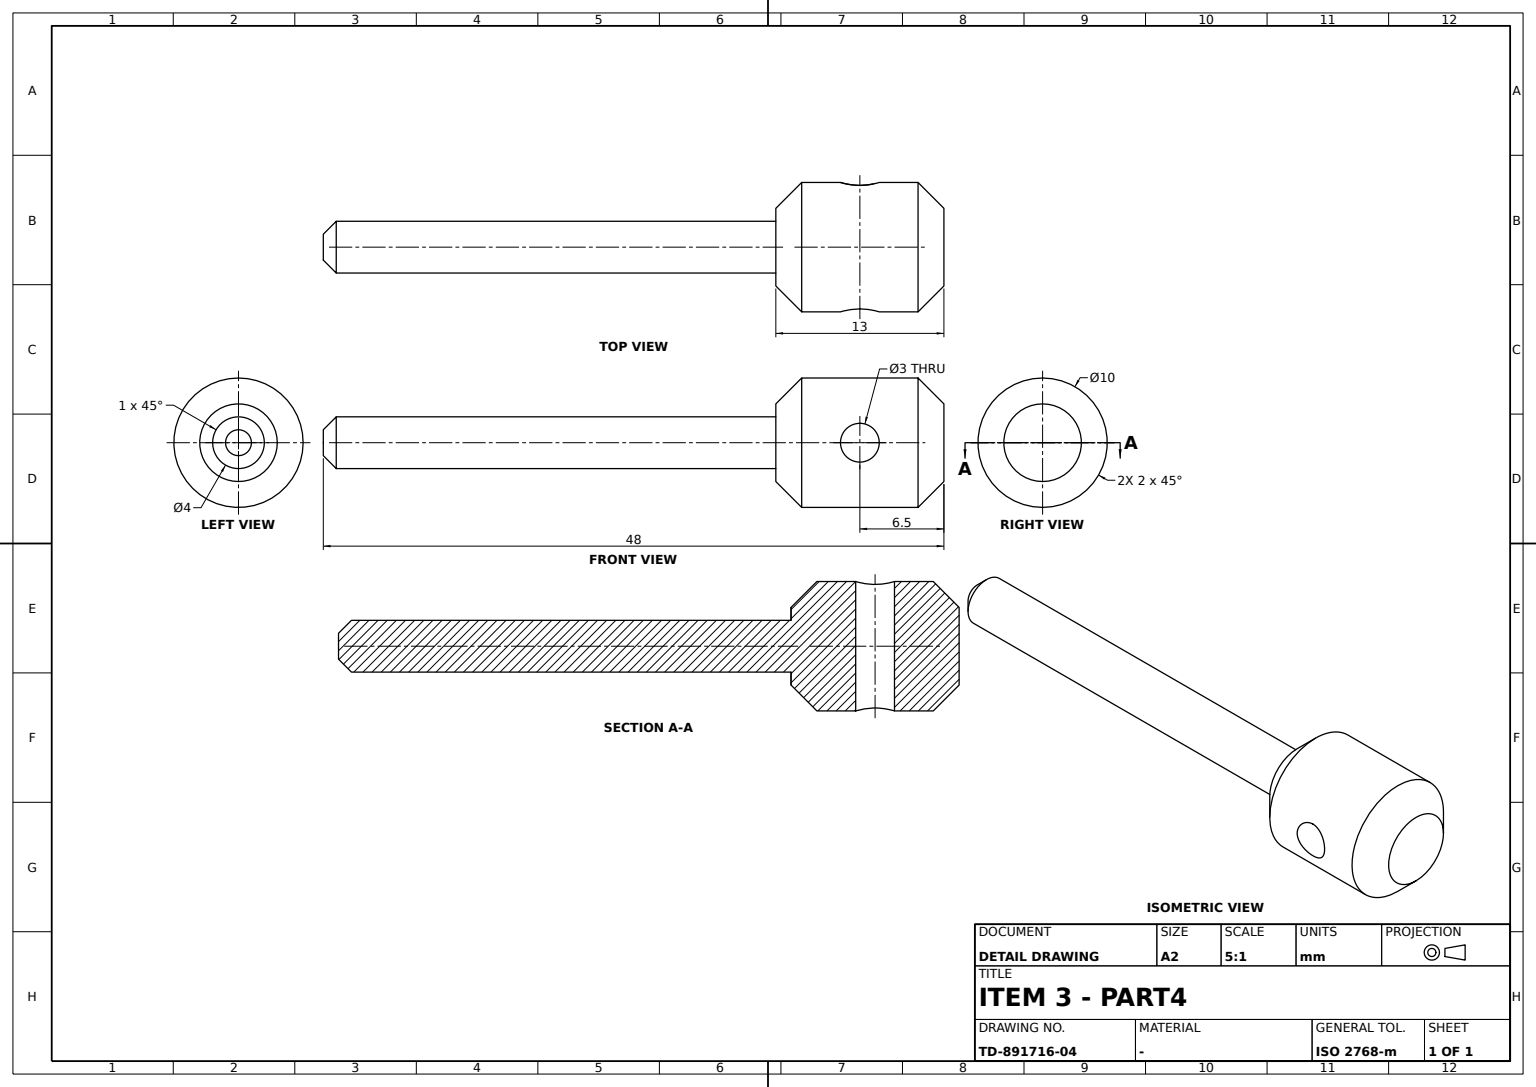
ISO-10303-21;
HEADER;
FILE_DESCRIPTION((''),'2;1');
FILE_NAME('','',(''),(''),'','','');
FILE_SCHEMA(('AUTOMOTIVE_DESIGN'));
ENDSEC;
DATA;
#1=APPLICATION_CONTEXT('');
#2=PRODUCT_CONTEXT('',#1,'mechanical');
#3=PRODUCT('','','',(#2));
#4=PRODUCT_DEFINITION_FORMATION('','',#3);
#5=PRODUCT_DEFINITION_CONTEXT('',#1,'design');
#6=PRODUCT_DEFINITION('','',#4,#5);
#7=PRODUCT_DEFINITION_SHAPE('','',#6);
#8=(LENGTH_UNIT()NAMED_UNIT(*)SI_UNIT(.MILLI.,.METRE.));
#9=(NAMED_UNIT(*)PLANE_ANGLE_UNIT()SI_UNIT($,.RADIAN.));
#10=(NAMED_UNIT(*)SI_UNIT($,.STERADIAN.)SOLID_ANGLE_UNIT());
#11=UNCERTAINTY_MEASURE_WITH_UNIT(LENGTH_MEASURE(0.005),#8,'distance_accuracy_value','');
#12=(GEOMETRIC_REPRESENTATION_CONTEXT(3)GLOBAL_UNCERTAINTY_ASSIGNED_CONTEXT((#11))GLOBAL_UNIT_ASSIGNED_CONTEXT((#8,#9,#10))REPRESENTATION_CONTEXT('',''));
#13=CARTESIAN_POINT('',(0.,-5.,2.));
#14=VERTEX_POINT('',#13);
#15=CARTESIAN_POINT('',(0.,0.,2.));
#16=DIRECTION('',(0.,0.,1.));
#17=DIRECTION('',(0.,-1.,0.));
#18=AXIS2_PLACEMENT_3D('',#15,#16,#17);
#19=CIRCLE('',#18,5.);
#20=EDGE_CURVE('',#14,#14,#19,.T.);
#21=ORIENTED_EDGE('',*,*,#20,.T.);
#22=EDGE_LOOP('',(#21));
#23=FACE_BOUND('',#22,.T.);
#24=CARTESIAN_POINT('',(-5.,0.,11.));
#25=VERTEX_POINT('',#24);
#26=CARTESIAN_POINT('',(0.,0.,11.));
#27=DIRECTION('',(0.,0.,-1.));
#28=DIRECTION('',(-1.,0.,0.));
#29=AXIS2_PLACEMENT_3D('',#26,#27,#28);
#30=CIRCLE('',#29,5.);
#31=EDGE_CURVE('',#25,#25,#30,.F.);
#32=ORIENTED_EDGE('',*,*,#31,.F.);
#33=EDGE_LOOP('',(#32));
#34=FACE_BOUND('',#33,.T.);
#35=CARTESIAN_POINT('',(-1.5,-4.769696,6.5));
#36=VERTEX_POINT('',#35);
#37=CARTESIAN_POINT('',(-1.175074,-4.887685,7.676025));
#38=CARTESIAN_POINT('',(-1.6623,-4.710734,6.499812));
#39=CARTESIAN_POINT('',(-1.175726,-4.887553,5.324727));
#40=CARTESIAN_POINT('',(0.001317,-5.0563,4.837246));
#41=CARTESIAN_POINT('',(1.176409,-4.887248,5.326292));
#42=CARTESIAN_POINT('',(1.66221,-4.71081,6.498832));
#43=CARTESIAN_POINT('',(1.174751,-4.887689,7.676372));
#44=CARTESIAN_POINT('',(0.000487,-5.056156,8.161901));
#45=B_SPLINE_CURVE_WITH_KNOTS('',3,(#37,#38,#39,#40,#41,#42,#43,#44,#37,#38,#39),.UNSPECIFIED.,.T.,.F.,(1,1,1,1,1,1,1,1,1,1,1,1,1,1,1),(-0.003536806,-0.00235787,-0.001178935,0.,0.001178935,0.00235787,0.003536806,0.004715741,0.005894676,0.007073611,0.008252547,0.009431482,0.010610417,0.011789352,0.012968288),.UNSPECIFIED.);
#46=EDGE_CURVE('',#36,#36,#45,.T.);
#47=ORIENTED_EDGE('',*,*,#46,.F.);
#48=EDGE_LOOP('',(#47));
#49=FACE_BOUND('',#48,.T.);
#50=CARTESIAN_POINT('',(0.,5.,5.));
#51=VERTEX_POINT('',#50);
#52=CARTESIAN_POINT('',(1.175321,4.887552,7.67551));
#53=CARTESIAN_POINT('',(1.662206,4.710787,6.499572));
#54=CARTESIAN_POINT('',(1.175856,4.887476,5.325056));
#55=CARTESIAN_POINT('',(-0.000283,5.056239,4.837629));
#56=CARTESIAN_POINT('',(-1.175299,4.887567,5.324429));
#57=CARTESIAN_POINT('',(-1.662217,4.710779,6.500428));
#58=CARTESIAN_POINT('',(-1.175833,4.887491,7.675005));
#59=CARTESIAN_POINT('',(0.000448,5.056239,8.162371));
#60=B_SPLINE_CURVE_WITH_KNOTS('',3,(#52,#53,#54,#55,#56,#57,#58,#59,#52,#53,#54),.UNSPECIFIED.,.T.,.F.,(1,1,1,1,1,1,1,1,1,1,1,1,1,1,1),(0.001178646,0.002357103,0.003535561,0.004714018,0.005892476,0.007070933,0.00824939,0.009427848,0.010606305,0.011784763,0.01296322,0.014141677,0.015320135,0.016498592,0.01767705),.UNSPECIFIED.);
#61=EDGE_CURVE('',#51,#51,#60,.T.);
#62=ORIENTED_EDGE('',*,*,#61,.F.);
#63=EDGE_LOOP('',(#62));
#64=FACE_BOUND('',#63,.T.);
#65=CARTESIAN_POINT('',(0.,0.,6.5));
#66=DIRECTION('',(0.,1.,0.));
#67=AXIS2_PLACEMENT_3D('',#65,#16,#66);
#68=CYLINDRICAL_SURFACE('',#67,5.);
#69=ADVANCED_FACE('',(#23,#34,#49,#64),#68,.T.);
#70=CARTESIAN_POINT('',(2.,0.,0.));
#71=VERTEX_POINT('',#70);
#72=CARTESIAN_POINT('',(0.,0.,0.));
#73=DIRECTION('',(1.,0.,0.));
#74=AXIS2_PLACEMENT_3D('',#72,#16,#73);
#75=CIRCLE('',#74,2.);
#76=EDGE_CURVE('',#71,#71,#75,.F.);
#77=ORIENTED_EDGE('',*,*,#76,.T.);
#78=EDGE_LOOP('',(#77));
#79=FACE_BOUND('',#78,.T.);
#80=CARTESIAN_POINT('',(0.,-2.,-34.));
#81=VERTEX_POINT('',#80);
#82=CARTESIAN_POINT('',(0.,0.,-34.));
#83=AXIS2_PLACEMENT_3D('',#82,#16,#17);
#84=CIRCLE('',#83,2.);
#85=EDGE_CURVE('',#81,#81,#84,.F.);
#86=ORIENTED_EDGE('',*,*,#85,.F.);
#87=EDGE_LOOP('',(#86));
#88=FACE_BOUND('',#87,.T.);
#89=CARTESIAN_POINT('',(0.,0.,-17.5));
#90=AXIS2_PLACEMENT_3D('',#89,#27,#17);
#91=CYLINDRICAL_SURFACE('',#90,2.);
#92=ADVANCED_FACE('',(#79,#88),#91,.T.);
#93=CARTESIAN_POINT('',(3.,0.,13.));
#94=VERTEX_POINT('',#93);
#95=CARTESIAN_POINT('',(0.,0.,13.));
#96=AXIS2_PLACEMENT_3D('',#95,#16,#73);
#97=CIRCLE('',#96,3.);
#98=EDGE_CURVE('',#94,#94,#97,.T.);
#99=ORIENTED_EDGE('',*,*,#98,.T.);
#100=EDGE_LOOP('',(#99));
#101=FACE_BOUND('',#100,.T.);
#102=AXIS2_PLACEMENT_3D('',#95,#16,#66);
#103=PLANE('',#102);
#104=ADVANCED_FACE('',(#101),#103,.T.);
#105=CARTESIAN_POINT('',(3.,0.,0.));
#106=VERTEX_POINT('',#105);
#107=CIRCLE('',#74,3.);
#108=EDGE_CURVE('',#106,#106,#107,.T.);
#109=ORIENTED_EDGE('',*,*,#108,.T.);
#110=EDGE_LOOP('',(#109));
#111=FACE_BOUND('',#110,.T.);
#112=ORIENTED_EDGE('',*,*,#20,.F.);
#113=EDGE_LOOP('',(#112));
#114=FACE_BOUND('',#113,.T.);
#115=CARTESIAN_POINT('',(0.,0.,-3.));
#116=DIRECTION('',(-0.044304636,-0.999018068,0.));
#117=AXIS2_PLACEMENT_3D('',#115,#16,#116);
#118=CONICAL_SURFACE('',#117,0.,0.785398163);
#119=ADVANCED_FACE('',(#111,#114),#118,.T.);
#120=ORIENTED_EDGE('',*,*,#46,.T.);
#121=EDGE_LOOP('',(#120));
#122=FACE_BOUND('',#121,.T.);
#123=ORIENTED_EDGE('',*,*,#61,.T.);
#124=EDGE_LOOP('',(#123));
#125=FACE_BOUND('',#124,.T.);
#126=AXIS2_PLACEMENT_3D('',#65,#66,#28);
#127=CYLINDRICAL_SURFACE('',#126,1.5);
#128=ADVANCED_FACE('',(#122,#125),#127,.F.);
#129=ORIENTED_EDGE('',*,*,#108,.F.);
#130=EDGE_LOOP('',(#129));
#131=FACE_BOUND('',#130,.T.);
#132=ORIENTED_EDGE('',*,*,#76,.F.);
#133=EDGE_LOOP('',(#132));
#134=FACE_BOUND('',#133,.T.);
#135=AXIS2_PLACEMENT_3D('',#72,#16,#66);
#136=PLANE('',#135);
#137=ADVANCED_FACE('',(#131,#134),#136,.F.);
#138=ORIENTED_EDGE('',*,*,#31,.T.);
#139=EDGE_LOOP('',(#138));
#140=FACE_BOUND('',#139,.T.);
#141=ORIENTED_EDGE('',*,*,#98,.F.);
#142=EDGE_LOOP('',(#141));
#143=FACE_BOUND('',#142,.T.);
#144=CARTESIAN_POINT('',(0.,0.,16.));
#145=DIRECTION('',(0.334252813,0.942483452,0.));
#146=AXIS2_PLACEMENT_3D('',#144,#27,#145);
#147=CONICAL_SURFACE('',#146,0.,0.785398163);
#148=ADVANCED_FACE('',(#140,#143),#147,.T.);
#149=ORIENTED_EDGE('',*,*,#85,.T.);
#150=EDGE_LOOP('',(#149));
#151=FACE_BOUND('',#150,.T.);
#152=CARTESIAN_POINT('',(-1.,0.,-35.));
#153=VERTEX_POINT('',#152);
#154=CARTESIAN_POINT('',(0.,0.,-35.));
#155=AXIS2_PLACEMENT_3D('',#154,#27,#28);
#156=CIRCLE('',#155,1.);
#157=EDGE_CURVE('',#153,#153,#156,.T.);
#158=ORIENTED_EDGE('',*,*,#157,.F.);
#159=EDGE_LOOP('',(#158));
#160=FACE_BOUND('',#159,.T.);
#161=CARTESIAN_POINT('',(0.,0.,-36.));
#162=DIRECTION('',(0.327950333,-0.944694966,0.));
#163=AXIS2_PLACEMENT_3D('',#161,#16,#162);
#164=CONICAL_SURFACE('',#163,0.,0.785398163);
#165=ADVANCED_FACE('',(#151,#160),#164,.T.);
#166=ORIENTED_EDGE('',*,*,#157,.T.);
#167=EDGE_LOOP('',(#166));
#168=FACE_BOUND('',#167,.T.);
#169=AXIS2_PLACEMENT_3D('',#154,#27,#17);
#170=PLANE('',#169);
#171=ADVANCED_FACE('',(#168),#170,.T.);
#172=CLOSED_SHELL('',(#69,#92,#104,#119,#128,#137,#148,#165,#171));
#173=MANIFOLD_SOLID_BREP('',#172);
#174=ADVANCED_BREP_SHAPE_REPRESENTATION('',(#173),#12);
#175=SHAPE_DEFINITION_REPRESENTATION(#7,#174);
ENDSEC;
END-ISO-10303-21;
